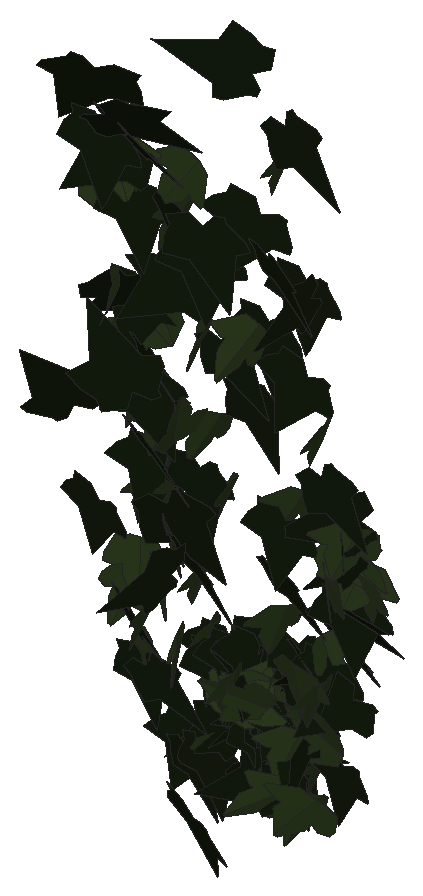
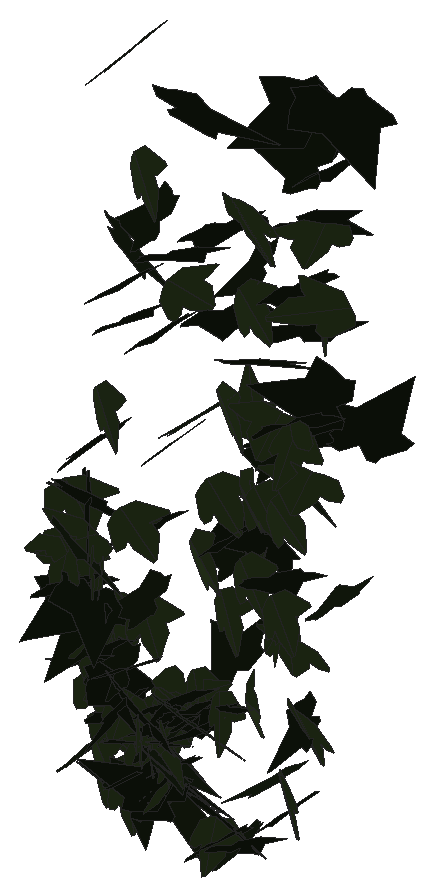
# SketchUp Ruby script. Lengths in inches.
U = 1.inch
M = Sketchup.active_model
def pt(a) = Geom::Point3d.new(a.map { |v| v * U })
def face(e, loops, mat)
  f = e.add_face(loops[0].map { |a| pt(a) })
  loops[1..].each { |l| e.add_face(l.map { |a| pt(a) }).erase! }
  f.material = f.back_material = mat if mat
  f
end
# faces: each face lists its corners as indices into pts; further lists are holes
def faces(e, pts, list, mat = nil) = list.each { |f| face(e, (f[0].is_a?(Array) ? f : [f]).map { |l| l.map { |i| pts[i] } }, mat) }
# xy, xz, yz: faces in a plane at the given z, y or x. An outline is a flat list of corners, or four numbers for a rectangle; further outlines are holes
def ring(l) = l.size == 4 ? [[l[0], l[1]], [l[2], l[1]], [l[2], l[3]], [l[0], l[3]]] : l.each_slice(2).to_a
def flat(e, list, mat, &to3) = list.each { |f| face(e, (f[0].is_a?(Array) ? f : [f]).map { |l| ring(l).map { |u, v| to3.(u, v) } }, mat) }
def xy(e, z, list, mat = nil) = flat(e, list, mat) { |x, y| [x, y, z] }
def xz(e, y, list, mat = nil) = flat(e, list, mat) { |x, z| [x, y, z] }
def yz(e, x, list, mat = nil) = flat(e, list, mat) { |y, z| [x, y, z] }
def lines(e, pts, list) = list.each { |a, b| e.add_line(pt(pts[a]), pt(pts[b])) }
# prism: a flat outline (further loops are holes) pulled along v
def prism(e, loops, v, mat = nil)
  f = face(e, loops, mat); d = Geom::Vector3d.new(v.map { |x| x * U })
  f.pushpull(f.normal.samedirection?(d) ? d.length : -d.length)
end
def box(e, o, s, mat = nil) = prism(e, [[o, [o[0] + s[0], o[1], o[2]], [o[0] + s[0], o[1] + s[1], o[2]], [o[0], o[1] + s[1], o[2]]]], [0, 0, s[2]], mat)
def at(x, y, z, deg = 0) = Geom::Transformation.translation(pt([x, y, z])) * Geom::Transformation.rotation(ORIGIN, Z_AXIS, deg.degrees)
def axes(o, x, y, z) = Geom::Transformation.new([*x, 0, *y, 0, *z, 0, *pt(o).to_a, 1])
def part(name) = M.definitions.add(name)
# library, detail: a bought-in or finely detailed component or shape, given as its bounding box
def library(name, o, s) = part(name).tap { |d| box(d.entities, o, s) }
def detail(e, o, s) = box(e.add_group.entities, o, s)
def put(e, d, t, mat = nil) = e.add_instance(d, t).tap { |i| i.material = mat if mat }
def group(e, t, mat = nil) = e.add_group.tap { |g| g.transformation = t; g.material = mat if mat }.entities
root = M.entities
M.materials.add("1026 AP 7946 SUNNY SIDE UP").color = [254, 231, 186]
M.materials.add("efeu1").color = [18, 25, 13]
M.materials.add("efeu2").color = [43, 57, 29]
c1 = part("ivyleaf_10")
p = [[0,0.5,-0.03],[-0.0625,2.02,-0.43],[-0.19,2.01,-0.46],[-0.54,1.05,-0.29],[-0.52,0.625,-0.18],[-0.83,0.76,-0.28],
  [-1.16,0.64,-0.33],[-1.15,0.33,-0.24],[-0.77,-0.39,0.02],[-0.3,-0.51,0.16],[0.04,-0.48,0.23],[-0.02,2.01,-0.4375],
  [-0.06,2.01,-0.43],[0.04,-0.49,0.23],[0.67,-0.49,0.14],[1.38,0.36,-0.2],[1.375,0.51,-0.24],[0.81,0.65,-0.19],
  [0.62,0.59,-0.15],[0.6,1.09,-0.28],[0.5,1.23,-0.31]]
faces(c1.entities,p,[[0,1,2,3,4,5,6,7,8,9,10],[11,12,0,13,14,15,16,17,18,19,20]],"efeu2")
c2 = part("ivyleaf_9")
p = [[1.54,2.16,1.25],[1.36,2.04,1.19],[-0.21,0.99,0.68],[-0.71,1.11,0.82],[-0.85,0.86,0.67],[-0.8,0.17,0.21],
  [-0.9,-0.01,0.1],[-0.67,-0.16,-0.02],[-0.08,-0.08,-0.05],[-0.03,-0.6,-0.4],[0.65,-0.88,-0.66],[0.83,-0.6,-0.49],
  [1.29,-0.42,-0.43],[1.8125,-0.07,-0.26],[1.21,0.44,0.15]]
faces(c2.entities,p,[[0,1,2,3,4,5,6,7,8,9,10,11,12,13,14]],"efeu1")
put(root,c1,axes([105.7,212.78,285.58],[0.45918,0.14187,0.10032],[0.12874,0.05236,-0.33397],[-0.23717,0.30309,0.01294]),"1026 AP 7946 SUNNY SIDE UP")
put(root,c1,axes([105.88,212.66,281.74],[0.43417,-0.19485,0.01464],[-0.00464,-0.03066,-0.34724],[0.30729,0.27484,-0.02592]),"1026 AP 7946 SUNNY SIDE UP")
put(root,c1,axes([105.59,212.39,288.06],[0.1643,0.04092,0.33482],[0.33547,0.25005,-0.10171],[-0.39038,0.2321,0.05352]),"1026 AP 7946 SUNNY SIDE UP")
put(root,c2,axes([106.09,211.16,285.3],[0.21858,0.08141,0.35047],[-0.50149,-0.11968,0.16328],[0.22422,-0.34702,0.02353]),"1026 AP 7946 SUNNY SIDE UP")
put(root,c1,axes([105.9375,212.79,286.09],[-0.13901,-0.27811,-0.18295],[0.1118,0.16181,-0.29923],[0.5053,-0.11231,0.01587]),"1026 AP 7946 SUNNY SIDE UP")
put(root,c2,axes([105.84,212.05,283.25],[-0.08146,-0.26994,0.18486],[0.03992,-0.18606,-0.27951],[0.50946,-0.02858,0.05146]),"1026 AP 7946 SUNNY SIDE UP")
put(root,c1,axes([106.09,212.79,280.69],[0.2514,-0.26095,-0.09253],[-0.0463,0.08536,-0.31419],[0.43071,0.16149,0.02023]),"1026 AP 7946 SUNNY SIDE UP")
put(root,c2,axes([105.77,212.1875,286.42],[0.15041,0.01967,0.34203],[0.44458,0.17689,-0.09371],[-0.27505,0.29667,0.03556]),"1026 AP 7946 SUNNY SIDE UP")
put(root,c2,axes([106.02,212.8,286.31],[-0.22858,-0.30858,0.01561],[0.00111,-0.01901,-0.3514],[0.48594,-0.14511,0.00814]),"1026 AP 7946 SUNNY SIDE UP")
put(root,c2,axes([105.96,212.89,280.42],[0.03832,-0.31386,0.02143],[-0.00963,-0.02312,-0.32434],[0.49469,0.02386,-0.00797]),"1026 AP 7946 SUNNY SIDE UP")
put(root,c1,axes([106.17,212.8,284.9],[0.00966,-0.30522,0.14236],[0.00404,-0.1399,-0.31532],[0.52794,0.00666,-0.00019]),"1026 AP 7946 SUNNY SIDE UP")
put(root,c2,axes([106.3,211.375,290.55],[0.26904,0.19511,-0.2779],[-0.24017,-0.22488,-0.26759],[-0.46672,0.22819,-0.02249]),"1026 AP 7946 SUNNY SIDE UP")
put(root,c1,axes([106.19,212.83,283.42],[-0.04911,-0.32425,0.05122],[0.00228,-0.05193,-0.33583],[0.51625,-0.03062,0.00635]),"1026 AP 7946 SUNNY SIDE UP")
put(root,c2,axes([106.03,212.36,281.58],[0.39116,-0.15109,-0.15529],[-0.20678,0.07215,-0.29936],[0.26311,0.28133,-0.00439]),"1026 AP 7946 SUNNY SIDE UP")
put(root,c2,axes([106.34,212.09,289.01],[-0.3762,-0.20301,0.16394],[-0.16861,-0.12086,-0.32328],[0.37013,-0.2614,0.01936]),"1026 AP 7946 SUNNY SIDE UP")
put(root,c1,axes([106.07,212.05,288.95],[0.34558,0.26649,0.06076],[0.08161,0.03156,-0.35509],[-0.42082,0.22496,-0.01897]),"1026 AP 7946 SUNNY SIDE UP")
put(root,c1,axes([106.1875,212.83,286.32],[0.49502,0.07598,0.11499],[0.14008,0.09453,-0.32583],[-0.1588,0.32021,0.07105]),"1026 AP 7946 SUNNY SIDE UP")
put(root,c2,axes([106.35,212.79,283.8125],[-0.26681,-0.28288,0.02221],[0.00793,-0.02999,-0.3394],[0.44622,-0.16861,0.01931]),"1026 AP 7946 SUNNY SIDE UP")
put(root,c2,axes([106.29,212.33,288.14],[-0.07052,-0.34068,-0.02926],[-0.00533,0.02714,-0.35377],[0.53728,-0.04444,-0.00735]),"1026 AP 7946 SUNNY SIDE UP")
put(root,c1,axes([106.36,212.27,282.57],[0.50019,-0.02307,0.08977],[0.13069,-0.04981,-0.32599],[0.05536,0.32608,-0.04148]),"1026 AP 7946 SUNNY SIDE UP")
put(root,c2,axes([106.38,211.5,289.55],[-0.1003,-0.3566,0.05564],[0.00714,-0.05769,-0.37323],[0.56755,-0.06229,0.01453]),"1026 AP 7946 SUNNY SIDE UP")
put(root,c2,axes([106.4,212.49,280.6],[0.24748,-0.25945,-0.10428],[0.02693,0.12346,-0.30226],[0.43624,0.13956,0.07781]),"1026 AP 7946 SUNNY SIDE UP")
put(root,c1,axes([106.73,212.5,284.78],[-0.11773,-0.30582,0.11071],[0.01038,-0.11348,-0.32339],[0.5105,-0.06822,0.03211]),"1026 AP 7946 SUNNY SIDE UP")
put(root,c1,axes([106.77,211.23,287.3],[0.13571,-0.28858,-0.17475],[-0.06163,0.16356,-0.30924],[0.52142,0.09444,0.00893]),"1026 AP 7946 SUNNY SIDE UP")
put(root,c2,axes([106.41,212.48,285.58],[0.24604,-0.27521,0.1194],[0.05577,-0.11456,-0.32586],[0.4672,0.15861,-0.02398]),"1026 AP 7946 SUNNY SIDE UP")
put(root,c1,axes([106.75,212.78,287.95],[0.01024,-0.32685,0.12016],[0.00502,-0.11846,-0.33748],[0.54665,0.00721,0.00085]),"1026 AP 7946 SUNNY SIDE UP")
put(root,c1,axes([106.83,212.69,283.7],[-0.0097,-0.32642,0.05331],[-0.00612,-0.05353,-0.33664],[0.52011,-0.00672,-0.00297]),"1026 AP 7946 SUNNY SIDE UP")
put(root,c2,axes([106.94,212.59,286.875],[-0.45266,-0.14819,0.11653],[-0.06223,-0.15618,-0.31316],[0.28728,-0.26734,0.11577]),"1026 AP 7946 SUNNY SIDE UP")
put(root,c2,axes([106.66,211.93,285.51],[-0.04964,-0.31532,-0.16787],[0.09427,0.1547,-0.32302],[0.54878,-0.0551,0.0403]),"1026 AP 7946 SUNNY SIDE UP")
put(root,c2,axes([106.89,212.9,279.57],[-0.25324,-0.26125,0.05394],[0.01754,-0.06943,-0.31312],[0.41906,-0.15497,0.0457]),"1026 AP 7946 SUNNY SIDE UP")
put(root,c1,axes([106.84,212.08,282.56],[-0.26571,0.23725,-0.16837],[0.08031,-0.16336,-0.29722],[-0.44705,-0.17036,0.04668]),"1026 AP 7946 SUNNY SIDE UP")
put(root,c2,axes([106.53,211.62,289.61],[0.28272,-0.21931,0.21087],[0.22883,-0.14657,-0.29255],[0.41401,0.23077,0.0177]),"1026 AP 7946 SUNNY SIDE UP")
put(root,c2,axes([106.625,212.04,284.53],[0.27203,-0.24924,0.14324],[0.09542,-0.12844,-0.31255],[0.43962,0.1821,-0.02079]),"1026 AP 7946 SUNNY SIDE UP")
put(root,c1,axes([106.94,212.54,284.8],[0.25121,-0.26639,0.16316],[0.11564,-0.14225,-0.3207],[0.47464,0.17565,-0.00822]),"1026 AP 7946 SUNNY SIDE UP")
put(root,c2,axes([106.78,211.15,290.09],[0.50375,0.13163,0.16447],[0.2455,0.03723,-0.35583],[-0.21213,0.35567,-0.02123]),"1026 AP 7946 SUNNY SIDE UP")
put(root,c1,axes([107.26,212.26,288.93],[0.45089,-0.18313,-0.11559],[-0.16181,0.04515,-0.34984],[0.29544,0.30421,-0.0152]),"1026 AP 7946 SUNNY SIDE UP")
put(root,c1,axes([107.2,211.47,282.34],[0.14485,-0.33855,0.05987],[0.01148,-0.06021,-0.3617],[0.54053,0.092,-0.00836]),"1026 AP 7946 SUNNY SIDE UP")
put(root,c1,axes([107.21,212.68,286.17],[0.18283,-0.31931,0.00937],[-0.00746,-0.01333,-0.35004],[0.50233,0.11602,-0.00861]),"1026 AP 7946 SUNNY SIDE UP")
put(root,c2,axes([106.92,212.28,288.1875],[0.33523,-0.2825,-0.0303],[-0.05627,0.00776,-0.36373],[0.44279,0.21486,-0.02328]),"1026 AP 7946 SUNNY SIDE UP")
put(root,c2,axes([106.98,212.64,279.42],[0.15994,-0.29435,0.03645],[0.004,-0.0383,-0.32089],[0.46647,0.10125,-0.00974]),"1026 AP 7946 SUNNY SIDE UP")
put(root,c1,axes([107.07,212.29,281.4],[0.1825,-0.16925,0.26901],[0.23928,-0.21341,-0.21265],[0.42826,0.19136,0.00417]),"1026 AP 7946 SUNNY SIDE UP")
put(root,c2,axes([107.5,210.67,286.24],[-0.44854,-0.23996,0.13288],[0.12766,0.10545,0.38364],[-0.40997,0.29537,-0.02592]),"1026 AP 7946 SUNNY SIDE UP")
put(root,c1,axes([107.36,212.7,284.76],[-0.12346,-0.30132,0.12438],[-0.03203,-0.12116,-0.32132],[0.51041,-0.08048,0.00992]),"1026 AP 7946 SUNNY SIDE UP")
put(root,c1,axes([107.3,212.65,281.46],[-0.0121,-0.30281,-0.1126],[0.03864,0.10675,-0.31071],[0.50382,-0.01546,0.02112]),"1026 AP 7946 SUNNY SIDE UP")
put(root,c1,axes([107.27,212.83,279.64],[-0.16696,-0.28131,-0.09495],[0.09702,0.07301,-0.30772],[0.45444,-0.11894,0.03081]),"1026 AP 7946 SUNNY SIDE UP")
put(root,c2,axes([107.54,212.82,279.95],[-0.47084,0.08828,-0.01075],[0.0032,-0.0316,-0.32033],[-0.13984,-0.29797,0.02887]),"1026 AP 7946 SUNNY SIDE UP")
put(root,c1,axes([107.34,211.76,283.44],[-0.30576,0.29605,0.05943],[-0.0768,0.0348,-0.36402],[-0.4675,-0.19935,0.02093]),"1026 AP 7946 SUNNY SIDE UP")
put(root,c2,axes([107.23,212.81,279.46],[-0.01069,-0.31327,-0.00158],[0.00075,-0.00025,-0.32281],[0.49259,-0.0068,0.00046]),"1026 AP 7946 SUNNY SIDE UP")
put(root,c2,axes([107.31,212.6,287.51],[-0.17544,-0.32342,-0.05284],[0.03044,0.04564,-0.35217],[0.51356,-0.11319,0.00282]),"1026 AP 7946 SUNNY SIDE UP")
put(root,c2,axes([107.26,212.54,284.02],[0.00138,-0.32937,0.02749],[0.00004,-0.02856,-0.33948],[0.51984,0.00087,-0.00004]),"1026 AP 7946 SUNNY SIDE UP")
put(root,c2,axes([107.93,212.75,290.49],[-0.31418,0.10588,0.28602],[-0.42042,0.08024,-0.22979],[-0.20181,-0.33202,0.03343]),"1026 AP 7946 SUNNY SIDE UP")
put(root,c1,axes([107.58,212.2,282.73],[0.01991,-0.32666,-0.03613],[-0.01267,0.03292,-0.33651],[0.51613,0.01341,-0.00687]),"1026 AP 7946 SUNNY SIDE UP")
put(root,c1,axes([107.59,212.77,283.78],[0.18058,-0.31151,0.10814],[0.04369,-0.10348,-0.3425],[0.51592,0.1178,-0.00885]),"1026 AP 7946 SUNNY SIDE UP")
put(root,c2,axes([107.59,212.77,281.27],[-0.25007,-0.27023,0.0362],[-0.00691,-0.03991,-0.32282],[0.42876,-0.15825,0.01591]),"1026 AP 7946 SUNNY SIDE UP")
put(root,c2,axes([107.29,211.82,283.77],[-0.11415,-0.11584,-0.34185],[0.48527,0.13979,-0.11925],[0.26242,-0.30888,0.07181]),"1026 AP 7946 SUNNY SIDE UP")
put(root,c2,axes([108.02,212.92,281.33],[-0.43771,0.14827,0.04047],[-0.10381,-0.0442,-0.31718],[-0.21733,-0.27752,0.07001]),"1026 AP 7946 SUNNY SIDE UP")
put(root,c2,axes([107.6,212.61,281.17],[-0.10146,-0.31318,-0.02373],[0.01254,0.02005,-0.32927],[0.49342,-0.06491,0.00349]),"1026 AP 7946 SUNNY SIDE UP")
put(root,c2,axes([107.47,212.8,285.98],[0.16596,-0.31502,-0.07264],[0.02712,0.07773,-0.33929],[0.50626,0.0991,0.04199]),"1026 AP 7946 SUNNY SIDE UP")
put(root,c1,axes([107.6875,211.52,285.1875],[-0.06084,-0.34755,-0.1021],[-0.0258,-0.09589,0.35965],[-0.56684,0.04167,-0.00541]),"1026 AP 7946 SUNNY SIDE UP")
put(root,c2,axes([107.75,212.82,280.96],[-0.16679,-0.28337,0.10368],[-0.00786,-0.10673,-0.31069],[0.47363,-0.10156,0.03136]),"1026 AP 7946 SUNNY SIDE UP")
put(root,c2,axes([107.82,212.74,281.24],[-0.16986,-0.30198,0.01406],[0.00615,-0.01771,-0.33035],[0.4754,-0.10767,0.0093]),"1026 AP 7946 SUNNY SIDE UP")
put(root,c2,axes([107.8,212.83,281.05],[-0.01694,-0.291,0.17713],[-0.00079,-0.17366,-0.30096],[0.5328,-0.00951,0.00518]),"1026 AP 7946 SUNNY SIDE UP")
put(root,c2,axes([108.24,212.46,279.62],[-0.04857,0.29908,0.07954],[-0.11195,0.06692,-0.3027],[-0.47194,-0.04666,0.06362]),"1026 AP 7946 SUNNY SIDE UP")
put(root,c2,axes([108.22,212.84,280.5],[-0.38712,0.1159,-0.16512],[0.13195,-0.17158,-0.26053],[-0.28257,-0.2389,0.10456]),"1026 AP 7946 SUNNY SIDE UP")
put(root,c2,axes([107.86,211.87,288.34],[-0.03996,-0.35283,-0.10225],[0.0501,0.09498,-0.36303],[0.5733,-0.0329,0.0246]),"1026 AP 7946 SUNNY SIDE UP")
put(root,c2,axes([108.38,212.9,280.46],[-0.4176,0.16277,0.04203],[-0.08547,-0.01299,-0.31843],[-0.24927,-0.26824,0.03878]),"1026 AP 7946 SUNNY SIDE UP")
put(root,c2,axes([108.07,212.81,288.23],[-0.31837,-0.27251,0.07461],[0.01732,-0.09858,-0.34364],[0.44367,-0.1917,0.06695]),"1026 AP 7946 SUNNY SIDE UP")
put(root,c2,axes([107.76,211.625,283.26],[0.28775,-0.27909,0.12323],[0.07562,-0.11313,-0.34383],[0.47242,0.1881,-0.02002]),"1026 AP 7946 SUNNY SIDE UP")
put(root,c1,axes([108.08,212.87,280.06],[0.02948,0.27003,-0.16286],[-0.01512,-0.15934,-0.27978],[-0.493,0.02104,-0.00116]),"1026 AP 7946 SUNNY SIDE UP")
put(root,c1,axes([108.18,212.0625,281.24],[0.00612,-0.32033,-0.04626],[0.02037,0.0432,-0.32949],[0.50782,0.00213,0.01377]),"1026 AP 7946 SUNNY SIDE UP")
put(root,c2,axes([108.1,212.82,281.29],[-0.17877,-0.31339,0.06833],[-0.00997,-0.07005,-0.34337],[0.50418,-0.11251,0.01744]),"1026 AP 7946 SUNNY SIDE UP")
put(root,c2,axes([107.99,212.77,285.36],[0.09873,-0.3319,-0.01609],[-0.00272,0.01365,-0.34791],[0.52232,0.06281,0.00123]),"1026 AP 7946 SUNNY SIDE UP")
put(root,c2,axes([108.3,212.91,280.8125],[-0.09027,-0.05195,0.31483],[-0.25914,-0.25847,-0.0786],[0.41336,-0.17338,0.01948]),"1026 AP 7946 SUNNY SIDE UP")
put(root,c1,axes([108.52,212.17,280.92],[-0.2256,-0.04107,-0.29064],[-0.39218,-0.13438,0.15016],[-0.21641,0.28634,0.03086]),"1026 AP 7946 SUNNY SIDE UP")
put(root,c1,axes([108.4,212.53,281.01],[-0.35259,-0.17548,0.13784],[-0.0745,-0.14938,-0.28241],[0.33987,-0.21479,0.08109]),"1026 AP 7946 SUNNY SIDE UP")
put(root,c1,axes([108.18,212.91,280.52],[-0.44313,0.05954,-0.1296],[0.1726,-0.08078,-0.2924],[-0.13533,-0.298,0.05143]),"1026 AP 7946 SUNNY SIDE UP")
put(root,c1,axes([108.32,212.66,280.76],[-0.10225,-0.29153,-0.121],[0.05905,0.11017,-0.30682],[0.48969,-0.07416,0.01174]),"1026 AP 7946 SUNNY SIDE UP")
put(root,c1,axes([108.12,212.23,280.73],[0.49842,0.04976,-0.16031],[0.20405,0.13062,0.31553],[0.15677,-0.3282,0.09901]),"1026 AP 7946 SUNNY SIDE UP")
put(root,c1,axes([108.31,212.74,280.98],[0.23696,-0.28221,-0.00228],[0.04114,0.01467,-0.32805],[0.44184,0.14999,0.03177]),"1026 AP 7946 SUNNY SIDE UP")
put(root,c2,axes([108.66,210.06,283.93],[-0.45858,0.27607,-0.07051],[0.04333,-0.07239,-0.41272],[-0.44574,-0.29106,0.03243]),"1026 AP 7946 SUNNY SIDE UP")
put(root,c2,axes([108.24,212.7,280.14],[-0.03295,-0.31742,-0.00061],[0.00796,-0.00155,-0.32768],[0.49905,-0.02094,0.00519]),"1026 AP 7946 SUNNY SIDE UP")
put(root,c2,axes([108.2,212.88,280.04],[0.08325,-0.30507,0.05095],[-0.00013,-0.05194,-0.31916],[0.4864,0.0522,-0.0088]),"1026 AP 7946 SUNNY SIDE UP")
put(root,c1,axes([108.53,212.96,280.85],[-0.25539,0.26829,0.01804],[-0.1437,-0.03756,-0.30731],[-0.39743,-0.15883,0.09952]),"1026 AP 7946 SUNNY SIDE UP")
put(root,c1,axes([108.46,212.78,280.54],[0.22872,-0.27991,-0.00582],[0.00778,0.00715,-0.32483],[0.44011,0.14534,0.00877]),"1026 AP 7946 SUNNY SIDE UP")
put(root,c2,axes([108.13,212.91,279.93],[0.03943,0.03725,0.31932],[0.48824,0.02722,-0.02911],[-0.04767,0.30957,-0.03401]),"1026 AP 7946 SUNNY SIDE UP")
put(root,c1,axes([108.53,212.82,280.4],[-0.13092,-0.26485,0.14395],[-0.0198,-0.14335,-0.28543],[0.47154,-0.07955,0.02798]),"1026 AP 7946 SUNNY SIDE UP")
put(root,c2,axes([108.31,212.92,280.8125],[-0.19815,0.2259,0.18759],[0.16274,-0.14897,0.26518],[0.42486,0.16242,-0.01409]),"1026 AP 7946 SUNNY SIDE UP")
put(root,c2,axes([108.86,212.1875,279.81],[-0.47055,0.10299,0.08849],[-0.14078,0.00103,-0.32483],[-0.15621,-0.31118,0.0262]),"1026 AP 7946 SUNNY SIDE UP")
put(root,c2,axes([108.1,212.9,279.84],[0.19966,-0.01895,0.29375],[0.41664,-0.10937,-0.12963],[0.16875,0.29245,-0.02749]),"1026 AP 7946 SUNNY SIDE UP")
put(root,c1,axes([108.57,212.8,289.39],[0.06197,-0.35024,0.00139],[-0.00051,-0.0034,-0.36312],[0.55075,0.03941,-0.00049]),"1026 AP 7946 SUNNY SIDE UP")
put(root,c2,axes([108.57,212.92,280.57],[-0.34175,-0.22569,0.02011],[0.09022,-0.08268,-0.30692],[0.34477,-0.20208,0.10025]),"1026 AP 7946 SUNNY SIDE UP")
put(root,c2,axes([108.42,212.95,280.15],[0.05233,-0.29092,-0.11194],[0.01879,0.10875,-0.30011],[0.48705,0.02706,0.02361]),"1026 AP 7946 SUNNY SIDE UP")
put(root,c1,axes([108.71,212.88,283.93],[-0.15815,-0.2742,0.14608],[-0.04332,-0.1422,-0.30096],[0.48459,-0.1022,0.02077]),"1026 AP 7946 SUNNY SIDE UP")
put(root,c1,axes([108.68,212.95,279.86],[-0.1342,-0.29778,-0.02092],[0.00768,0.01796,-0.31901],[0.46907,-0.08549,-0.00076]),"1026 AP 7946 SUNNY SIDE UP")
put(root,c2,axes([108.47,212.54,286.76],[-0.02919,-0.3385,0.05691],[-0.00045,-0.05723,-0.34957],[0.5398,-0.01835,0.00279]),"1026 AP 7946 SUNNY SIDE UP")
put(root,c2,axes([108.4,212.86,280.61],[0.17242,-0.23538,0.18391],[0.0908,-0.17111,-0.26798],[0.45685,0.12284,-0.01615]),"1026 AP 7946 SUNNY SIDE UP")
put(root,c1,axes([108.73,211.77,287.02],[-0.15612,-0.21395,0.2933],[0.05329,-0.30107,-0.22173],[0.55898,-0.03105,0.10306]),"1026 AP 7946 SUNNY SIDE UP")
put(root,c1,axes([108.75,212.47,282.3],[-0.14439,-0.31042,0.04717],[0.00643,-0.05071,-0.33327],[0.49376,-0.09012,0.01813]),"1026 AP 7946 SUNNY SIDE UP")
put(root,c2,axes([108.85,212.55,279.72],[0.00382,0.30879,0.05124],[-0.00788,0.04802,-0.31779],[-0.4913,0.00163,0.00549]),"1026 AP 7946 SUNNY SIDE UP")
put(root,c2,axes([108.42,212.75,282.74],[0.30039,-0.25602,0.03658],[0.04475,-0.02486,-0.32913],[0.40426,0.19299,0.00926]),"1026 AP 7946 SUNNY SIDE UP")
put(root,c1,axes([108.7,212.45,279.95],[-0.11979,-0.20348,-0.25738],[0.20658,0.21351,-0.22019],[0.46109,-0.14852,0.03179]),"1026 AP 7946 SUNNY SIDE UP")
put(root,c1,axes([109,212.07,279.72],[-0.10356,-0.12353,0.30586],[-0.17345,-0.27676,-0.14512],[0.47605,-0.12771,0.01367]),"1026 AP 7946 SUNNY SIDE UP")
put(root,c2,axes([108.72,212.59,283.67],[-0.1199,-0.31338,0.0726],[-0.0086,-0.07298,-0.33247],[0.50561,-0.07555,0.01156]),"1026 AP 7946 SUNNY SIDE UP")
put(root,c1,axes([108.84,212.86,281.08],[-0.49306,0.02221,-0.04233],[0.0581,-0.05398,-0.31991],[-0.0452,-0.31163,0.05051]),"1026 AP 7946 SUNNY SIDE UP")
put(root,c2,axes([108.66,212.65,279.9],[0.10857,-0.30918,0.01069],[-0.00367,-0.01295,-0.3264],[0.48652,0.0689,-0.00485]),"1026 AP 7946 SUNNY SIDE UP")
put(root,c2,axes([108.75,212.88,281.1],[0.17964,-0.21459,-0.21044],[-0.14318,0.18153,-0.24936],[0.44192,0.14604,0.00475]),"1026 AP 7946 SUNNY SIDE UP")
put(root,c2,axes([109.03,212.77,281.38],[-0.03927,0.28073,-0.14441],[0.00679,-0.1419,-0.29108],[-0.49448,-0.02424,0.00747]),"1026 AP 7946 SUNNY SIDE UP")
put(root,c2,axes([108.78,212.85,281.61],[0.01213,-0.31573,-0.05198],[0.10132,0.04922,-0.31814],[0.492,-0.00235,0.0668]),"1026 AP 7946 SUNNY SIDE UP")
put(root,c1,axes([109.15,212.28,280.52],[-0.281,-0.22851,0.12313],[-0.01824,-0.13964,-0.29058],[0.40603,-0.16442,0.07216]),"1026 AP 7946 SUNNY SIDE UP")
put(root,c2,axes([108.9375,212.8,287.44],[-0.07423,-0.33189,0.07781],[0.01157,-0.07913,-0.34532],[0.53574,-0.04428,0.01824]),"1026 AP 7946 SUNNY SIDE UP")
put(root,c2,axes([109.1,212.5625,280.61],[-0.33603,-0.23072,-0.03353],[0.07615,-0.00258,-0.32174],[0.35809,-0.21596,0.03696]),"1026 AP 7946 SUNNY SIDE UP")
put(root,c2,axes([108.85,212.82,281.53],[0.3154,-0.23899,0.06329],[0.04009,-0.06043,-0.32119],[0.38647,0.20131,-0.01833]),"1026 AP 7946 SUNNY SIDE UP")
put(root,c2,axes([108.89,212.05,288.11],[0.24941,-0.28802,0.11869],[0.06302,-0.11114,-0.33891],[0.48466,0.16267,-0.01701]),"1026 AP 7946 SUNNY SIDE UP")
put(root,c2,axes([109.13,212.375,280.57],[-0.33425,-0.01444,-0.26206],[0.39681,-0.0568,-0.21433],[-0.05424,-0.32654,0.0469]),"1026 AP 7946 SUNNY SIDE UP")
put(root,c2,axes([109.34,212.875,282.55],[0.09992,0.31701,0.01457],[-0.01495,0.01449,-0.33276],[-0.49863,0.06309,0.0129]),"1026 AP 7946 SUNNY SIDE UP")
put(root,c1,axes([109.29,212.75,280.13],[0.08758,-0.31187,0.03396],[0.00111,-0.03515,-0.32652],[0.49341,0.05544,-0.00529]),"1026 AP 7946 SUNNY SIDE UP")
put(root,c1,axes([109.34,212.36,279.54],[-0.1112,-0.29123,0.14136],[-0.01995,-0.13954,-0.30896],[0.50693,-0.06937,0.01885]),"1026 AP 7946 SUNNY SIDE UP")
put(root,c1,axes([109.39,212.6,285.41],[0.07896,-0.33317,-0.01852],[-0.01221,0.01509,-0.34697],[0.52434,0.05052,-0.00529]),"1026 AP 7946 SUNNY SIDE UP")
put(root,c1,axes([109.4375,212.67,282.92],[-0.31538,0.24601,0.07024],[-0.12143,0.02234,-0.3236],[-0.38199,-0.21022,0.04488]),"1026 AP 7946 SUNNY SIDE UP")
put(root,c2,axes([109.53,212.09,287.71],[-0.44295,0.1479,-0.15913],[0.17628,-0.11702,-0.32497],[-0.28748,-0.29964,0.04592]),"1026 AP 7946 SUNNY SIDE UP")
put(root,c1,axes([109.3,212.79,281.8125],[0.03488,0.31548,0.02779],[0.01217,0.0247,-0.3256],[-0.49749,0.02272,-0.00602]),"1026 AP 7946 SUNNY SIDE UP")
put(root,c1,axes([109.52,212.7,283],[-0.24306,0.26529,0.11032],[-0.18369,0.05079,-0.30737],[-0.40967,-0.18017,0.07237]),"1026 AP 7946 SUNNY SIDE UP")
put(root,c1,axes([109.54,212.53,280.98],[-0.23696,-0.26532,0.08864],[-0.05093,-0.08221,-0.31458],[0.43635,-0.15367,0.01142]),"1026 AP 7946 SUNNY SIDE UP")
put(root,c1,axes([109.51,211.91,281.85],[-0.46772,0.12295,0.02595],[-0.04985,-0.01276,-0.33075],[-0.19073,-0.29819,0.0228]),"1026 AP 7946 SUNNY SIDE UP")
put(root,c2,axes([109.16,210.02,280.25],[0.05575,-0.26709,0.30639],[0.14117,-0.28718,-0.27699],[0.61431,0.09023,0.03585]),"1026 AP 7946 SUNNY SIDE UP")
put(root,c2,axes([109.44,212.14,286.42],[-0.21778,-0.27448,0.15281],[-0.03848,-0.15392,-0.31456],[0.49025,-0.13401,0.04319]),"1026 AP 7946 SUNNY SIDE UP")
put(root,c2,axes([109.82,212.8125,283.98],[-0.48466,0.06771,0.10753],[-0.17589,-0.03107,-0.32091],[-0.08446,-0.32381,0.05128]),"1026 AP 7946 SUNNY SIDE UP")
put(root,c2,axes([109.4375,212.73,281.5625],[-0.13074,-0.30059,0.0511],[-0.01033,-0.0514,-0.32151],[0.47937,-0.08309,0.00701]),"1026 AP 7946 SUNNY SIDE UP")
put(root,c1,axes([109.91,212.07,280.8],[-0.10743,0.0345,-0.33841],[-0.42711,0.18533,0.07929],[0.29602,0.27992,-0.0084]),"1026 AP 7946 SUNNY SIDE UP")
put(root,c2,axes([109.43,212.875,282.03],[0.44647,-0.06805,-0.13597],[-0.19478,0.04701,-0.30011],[0.12778,0.30941,0.01763]),"1026 AP 7946 SUNNY SIDE UP")
put(root,c2,axes([109.71,212.55,283.99],[0.16387,-0.08381,-0.31965],[-0.44987,0.12333,-0.1328],[0.22867,0.30271,-0.03219]),"1026 AP 7946 SUNNY SIDE UP")
put(root,c1,axes([109.83,211.74,279.94],[-0.42814,-0.05827,0.18938],[-0.25339,-0.10697,-0.28094],[0.16746,-0.31082,0.05908]),"1026 AP 7946 SUNNY SIDE UP")
put(root,c2,axes([109.84,212.84,283.39],[-0.37511,0.21816,-0.05021],[0.03866,-0.04706,-0.33279],[-0.34979,-0.23915,0.01706]),"1026 AP 7946 SUNNY SIDE UP")
put(root,c2,axes([109.44,211.75,290.53],[0.2495,-0.31813,-0.13898],[-0.06052,0.12926,-0.36479],[0.53885,0.16182,0.02338]),"1026 AP 7946 SUNNY SIDE UP")
put(root,c2,axes([109.57,212.8,279.99],[-0.04166,-0.27583,0.14383],[-0.00228,-0.14159,-0.28608],[0.48723,-0.02425,0.01096]),"1026 AP 7946 SUNNY SIDE UP")
put(root,c2,axes([109.48,212.84,282.4],[0.50813,0.01632,0.00002],[-0.00264,0.03166,-0.33155],[-0.02553,0.3216,0.03454]),"1026 AP 7946 SUNNY SIDE UP")
put(root,c2,axes([109.55,212.41,284.72],[0.16932,-0.29565,-0.12487],[-0.03108,0.11973,-0.32273],[0.50047,0.10746,0.0222]),"1026 AP 7946 SUNNY SIDE UP")
put(root,c2,axes([109.88,212.59,281.27],[-0.39335,-0.16566,0.11557],[-0.04974,-0.14599,-0.29316],[0.31148,-0.23251,0.09913]),"1026 AP 7946 SUNNY SIDE UP")
put(root,c1,axes([109.84,211.96,281.71],[-0.00176,-0.32715,-0.00113],[-0.00326,-0.00075,-0.33703],[0.5144,-0.00112,-0.00214]),"1026 AP 7946 SUNNY SIDE UP")
put(root,c1,axes([109.81,212.87,283.15],[0.46929,0.10664,-0.08118],[-0.11857,-0.02496,-0.32664],[-0.17219,0.30783,0.00366]),"1026 AP 7946 SUNNY SIDE UP")
put(root,c1,axes([109.91,212.625,283.85],[-0.31194,-0.23057,0.13439],[-0.03063,-0.15139,-0.30402],[0.41645,-0.18384,0.07831]),"1026 AP 7946 SUNNY SIDE UP")
put(root,c1,axes([109.86,212.89,282.98],[-0.41623,0.18675,0.02507],[-0.05551,-0.00982,-0.33252],[-0.29067,-0.26555,0.0276]),"1026 AP 7946 SUNNY SIDE UP")
put(root,c2,axes([109.73,212.875,282.59],[-0.15413,-0.30766,-0.03265],[0.02813,0.02572,-0.33237],[0.48524,-0.09922,0.0089]),"1026 AP 7946 SUNNY SIDE UP")
put(root,c1,axes([109.5,212.82,283.375],[0.31891,0.08287,0.25429],[0.34224,0.11668,-0.22434],[-0.22343,0.29701,0.01932]),"1026 AP 7946 SUNNY SIDE UP")
